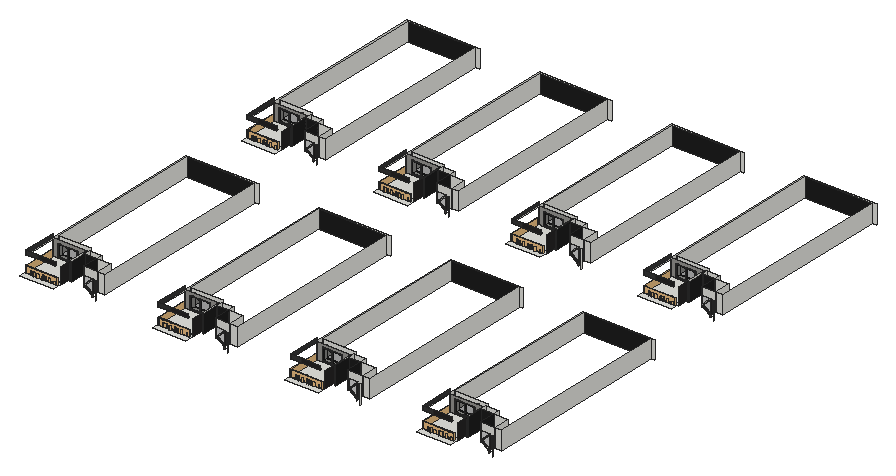
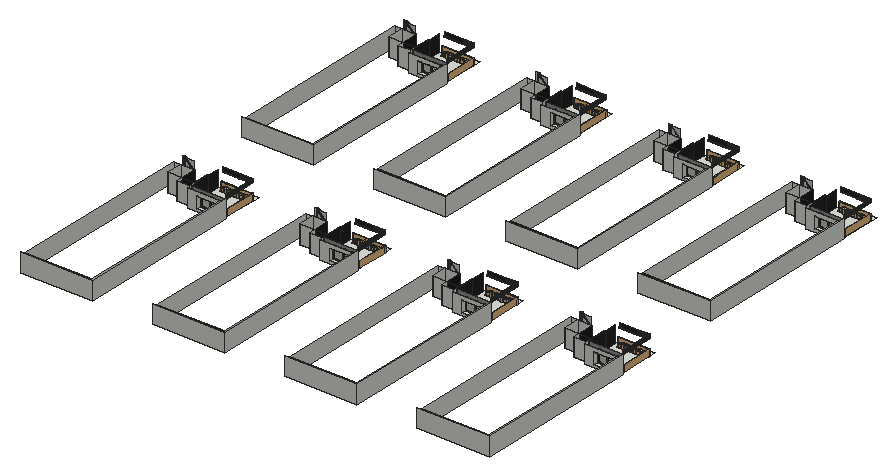
# SketchUp Ruby script. Lengths in inches.
U = 1.inch
M = Sketchup.active_model
def pt(a) = Geom::Point3d.new(a.map { |v| v * U })
def face(e, loops, mat)
  f = e.add_face(loops[0].map { |a| pt(a) })
  loops[1..].each { |l| e.add_face(l.map { |a| pt(a) }).erase! }
  f.material = f.back_material = mat if mat
  f
end
# faces: each face lists its corners as indices into pts; further lists are holes
def faces(e, pts, list, mat = nil) = list.each { |f| face(e, (f[0].is_a?(Array) ? f : [f]).map { |l| l.map { |i| pts[i] } }, mat) }
# xy, xz, yz: faces in a plane at the given z, y or x. An outline is a flat list of corners, or four numbers for a rectangle; further outlines are holes
def ring(l) = l.size == 4 ? [[l[0], l[1]], [l[2], l[1]], [l[2], l[3]], [l[0], l[3]]] : l.each_slice(2).to_a
def flat(e, list, mat, &to3) = list.each { |f| face(e, (f[0].is_a?(Array) ? f : [f]).map { |l| ring(l).map { |u, v| to3.(u, v) } }, mat) }
def xy(e, z, list, mat = nil) = flat(e, list, mat) { |x, y| [x, y, z] }
def xz(e, y, list, mat = nil) = flat(e, list, mat) { |x, z| [x, y, z] }
def yz(e, x, list, mat = nil) = flat(e, list, mat) { |y, z| [x, y, z] }
def lines(e, pts, list) = list.each { |a, b| e.add_line(pt(pts[a]), pt(pts[b])) }
# prism: a flat outline (further loops are holes) pulled along v
def prism(e, loops, v, mat = nil)
  f = face(e, loops, mat); d = Geom::Vector3d.new(v.map { |x| x * U })
  f.pushpull(f.normal.samedirection?(d) ? d.length : -d.length)
end
def box(e, o, s, mat = nil) = prism(e, [[o, [o[0] + s[0], o[1], o[2]], [o[0] + s[0], o[1] + s[1], o[2]], [o[0], o[1] + s[1], o[2]]]], [0, 0, s[2]], mat)
def at(x, y, z, deg = 0) = Geom::Transformation.translation(pt([x, y, z])) * Geom::Transformation.rotation(ORIGIN, Z_AXIS, deg.degrees)
def axes(o, x, y, z) = Geom::Transformation.new([*x, 0, *y, 0, *z, 0, *pt(o).to_a, 1])
def part(name) = M.definitions.add(name)
# library, detail: a bought-in or finely detailed component or shape, given as its bounding box
def library(name, o, s) = part(name).tap { |d| box(d.entities, o, s) }
def detail(e, o, s) = box(e.add_group.entities, o, s)
def put(e, d, t, mat = nil) = e.add_instance(d, t).tap { |i| i.material = mat if mat }
def group(e, t, mat = nil) = e.add_group.tap { |g| g.transformation = t; g.material = mat if mat }.entities
root = M.entities
M.materials.add("Glass_Tinted_Gray").color = [0, 0, 0]
M.materials["Glass_Tinted_Gray"].alpha = 0.125
M.materials.add("Material__1").color = [95, 70, 46]
M.materials.add("[0135_DarkGray]").color = [81, 81, 81]
M.materials.add("[Carrera Marble]").color = [207, 207, 207]
M.materials.add("[Color M06]").color = [86, 86, 86]
M.materials.add("[Color M08]").color = [30, 30, 30]
M.materials.add("[Field Square Tile]").color = [211, 167, 108]
M.materials.add("[Granite Dark Gray]").color = [38, 37, 37]
M.materials.add("[Granite Light Gray]").color = [149, 148, 144]
M.materials.add("[Granite Tile]1").color = [68, 65, 63]
M.materials.add("[Mirror 02]").color = [229, 229, 229]
M.materials.add("[Slate Light Tile]").color = [54, 54, 54]
M.materials.add("[Terrazzo Light Blue]").color = [196, 214, 227]
c1 = library("Areca palm plant",[0,0,0],[49.1,36.6,54.46])
c2 = library("Group\#74",[-84.69,-90.07,-0.36],[176.51,175.13,171.4])
c3 = library("Group38\#2",[14.01,28.44,-23.43],[18.58,18.32,38.89])
c4 = library("Group\#130",[-7.34,-1.2,0],[38.67,35.81,49.04])
c5 = library("Group20\#1",[-20.81,-17.08,3.79],[39.86,39.43,37.51])
c6 = part("Group\#3")
xy(c6.entities,0,[[0,0,6,234.8],[30,0,36,234.8]])
xy(c6.entities,3,[[6,0,30,234.8]])
xy(c6.entities,7,[[6,5,30,229.8]],"Material__1")
xy(c6.entities,15,[[[0,0,36,234.8],[6,5,30,229.8]]])
xz(c6.entities,0,[[0,0,6,0,6,3,30,3,30,0,36,0,36,15,0,15]])
xz(c6.entities,5,[[6,7,30,15]])
xz(c6.entities,229.8,[[6,7,30,15]])
xz(c6.entities,234.8,[[0,0,0,15,36,15,36,0,30,0,30,3,6,3,6,0]])
yz(c6.entities,0,[[0,0,234.8,15]])
yz(c6.entities,6,[[0,0,234.8,3],[5,7,229.8,15]])
yz(c6.entities,30,[[0,0,234.8,3],[5,7,229.8,15]])
yz(c6.entities,36,[[0,0,234.8,15]])
c7 = part("Group\#5")
put(c7.entities,c1,axes([-6.2,158.41,6.08],[0.45017,-0.56191,0],[0.66137,0.52986,0],[0,0,0.72]))
put(c7.entities,c1,axes([-6.2,56.6,6.08],[0.45017,-0.56191,0],[0.66137,0.52986,0],[0,0,0.72]))
put(c7.entities,c2,axes([17.19,15.79,6.07],[-0.08133,-0.14087,0],[0.14087,-0.08133,0],[0,0,0.1725]))
put(c7.entities,c2,axes([14.93,173.12,6.05],[-0.04961,-0.08593,0],[0.08593,-0.04961,0],[0,0,0.10522]))
put(c7.entities,c2,axes([17.19,223.04,6.07],[-0.08133,-0.14087,0],[0.14087,-0.08133,0],[0,0,0.1725]))
put(c7.entities,c3,axes([-4.1,-1.15,28.17],[0.8848,0,0],[0,0.94674,0],[0,0,0.85826]))
put(c7.entities,c2,axes([14.93,193.18,6.05],[-0.04961,-0.08593,0],[0.08593,-0.04961,0],[0,0,0.10522]))
put(c7.entities,c2,axes([14.93,91.37,6.05],[-0.04961,-0.08593,0],[0.08593,-0.04961,0],[0,0,0.10522]))
put(c7.entities,c4,axes([24.9375,191.72,8],[0,0.79,0],[-0.79,0,0],[0,0,0.79]))
put(c7.entities,c5,axes([18.97,181.79,4.77],[0,0.85,0],[-0.85,0,0],[0,0,0.85]))
put(c7.entities,c2,axes([14.93,145.87,6.05],[-0.04961,-0.08593,0],[0.08593,-0.04961,0],[0,0,0.10522]))
put(c7.entities,c5,axes([18.97,79.98,4.77],[0,0.85,0],[-0.85,0,0],[0,0,0.85]))
put(c7.entities,c2,axes([14.93,71.3,6.05],[-0.04961,-0.08593,0],[0.08593,-0.04961,0],[0,0,0.10522]))
put(c7.entities,c4,axes([24.9375,89.91,8],[0,0.79,0],[-0.79,0,0],[0,0,0.79]))
put(c7.entities,c2,axes([14.93,44.05,6.05],[-0.04961,-0.08593,0],[0.08593,-0.04961,0],[0,0,0.10522]))
put(c7.entities,c2,axes([17.19,121.23,6.07],[-0.08133,-0.14087,0],[0.14087,-0.08133,0],[0,0,0.1725]))
put(c7.entities,c6,at(0,0,0))
put(c7.entities,c3,axes([-4.1,100.66,28.17],[0.8848,0,0],[0,0.94674,0],[0,0,0.85826]))
c8 = library("Glass Railing",[0,0,0],[139.5,4.76,42])
c9 = part("PENTEK_RP Fineline 50S_Sliding_DoorCase_E1")
box(c9.entities,[0,0,0],[1.51,3.66,99.27],"[0135_DarkGray]")
c10 = part("PENTEK_RP Fineline 50S_SlidingDooe_Case_E2")
box(c10.entities,[0,0,0],[96.25,3.66,1.51],"[0135_DarkGray]")
c11 = part("pentek_RP Fineline 50S_SlidingDoor_Case")
put(c11.entities,c9,at(97.76,0,0))
put(c11.entities,c10,at(1.51,0,0))
put(c11.entities,c9,at(0,0,0))
put(c11.entities,c10,at(1.51,0,97.76))
c12 = part("PENTEK_RP Fineline 50S_SlidingDoor_GlazingBead_2")
box(c12.entities,[0,0,0],[0.56,0.59,94.39],"[0135_DarkGray]")
c13 = part("PENTEK_RP Fineline 50S_SlidingDoor_Glass")
box(c13.entities,[0,0,0],[46.58,0.16,94.39],"Glass_Tinted_Gray")
c14 = part("PENTEK_RP Fineline 50S_SlidingDoor_GlazingBead")
box(c14.entities,[0,0,0],[45.47,0.59,0.56],"[0135_DarkGray]")
c15 = part("PENTEK_RP Fineline 50S_SlidingDoor_Leaf_E1")
xy(c15.entities,0,[[0,0,0.93,1.97],[0.93,1.57,1.49,1.97]],"[0135_DarkGray]")
xy(c15.entities,96.25,[[0,0,0.93,0,0.93,1.57,1.49,1.57,1.49,1.97,0,1.97]],"[0135_DarkGray]")
xz(c15.entities,0,[[0,0,0.93,96.25]],"[0135_DarkGray]")
xz(c15.entities,1.57,[[0.93,0,1.49,95.32],[0.93,95.32,1.49,96.25]],"[0135_DarkGray]")
xz(c15.entities,1.97,[[0,0,1.49,96.25]],"[0135_DarkGray]")
yz(c15.entities,0,[[0,0,1.97,96.25]],"[0135_DarkGray]")
yz(c15.entities,0.93,[[0,0,1.57,0.93],[0,0.93,1.57,95.32],[0,95.32,1.57,96.25]],"[0135_DarkGray]")
yz(c15.entities,1.49,[[1.57,0,1.97,95.32],[1.57,95.32,1.97,96.25]],"[0135_DarkGray]")
c16 = part("PENTEK_RP Fineline 50S_SlidingDoor_Leaf_E2")
xy(c16.entities,0,[[0,0,0,1.57,0.56,1.57,0.56,1.97,46.02,1.97,46.02,1.57,46.58,1.57,46.58,0]],"[0135_DarkGray]")
xy(c16.entities,0.93,[[0,0,46.58,1.57]],"[0135_DarkGray]")
xy(c16.entities,1.49,[[0.56,1.57,46.02,1.97]],"[0135_DarkGray]")
xz(c16.entities,0,[[0,0,46.58,0.93]],"[0135_DarkGray]")
xz(c16.entities,1.57,[[0,0,0.56,0.93],[46.02,0,46.58,0.93],[0.56,0.93,46.02,1.49]],"[0135_DarkGray]")
xz(c16.entities,1.97,[[0.56,0,46.02,1.49]],"[0135_DarkGray]")
yz(c16.entities,0,[[0,0,1.57,0.93]],"[0135_DarkGray]")
yz(c16.entities,0.56,[[1.57,0,1.97,0.93],[1.57,0.93,1.97,1.49]],"[0135_DarkGray]")
yz(c16.entities,46.02,[[1.57,0,1.97,0.93],[1.57,0.93,1.97,1.49]],"[0135_DarkGray]")
yz(c16.entities,46.58,[[0,0,1.57,0.93]],"[0135_DarkGray]")
c17 = part("PENTEK_RP Fineline S_SlidingDoor_Leaf1")
put(c17.entities,c12,at(0.93,0,0.93))
put(c17.entities,c12,at(46.96,0,0.93))
put(c17.entities,c13,at(1.49,1.42,0.93))
put(c17.entities,c14,at(1.49,0,0.93))
put(c17.entities,c13,at(1.49,0.59,0.93),"[Terrazzo Light Blue]")
put(c17.entities,c15,at(0,0,0))
put(c17.entities,c15,axes([48.44,0,0],[-1,0,0],[0,1,0],[0,0,1]))
put(c17.entities,c16,axes([0.93,0,96.25],[1,0,0],[0,1,0],[0,0,-1]))
put(c17.entities,c16,at(0.93,0,0))
put(c17.entities,c14,at(1.49,0,94.77))
c18 = part("PENTEK_RP Fineline 50S_SlidingDoor_Leaf2")
put(c18.entities,c13,at(1.49,1.42,0.93))
put(c18.entities,c14,at(1.49,0,94.77))
put(c18.entities,c12,at(46.96,0,0.93))
put(c18.entities,c13,at(1.49,0.59,0.93),"[Mirror 02]")
put(c18.entities,c12,at(0.93,0,0.93))
put(c18.entities,c15,at(0,0,0))
put(c18.entities,c15,axes([48.44,0,0],[-1,0,0],[0,1,0],[0,0,1]))
put(c18.entities,c14,at(1.49,0,0.93))
put(c18.entities,c16,axes([0.93,0,96.25],[1,0,0],[0,1,0],[0,0,-1]))
put(c18.entities,c16,at(0.93,0,0))
c19 = part("PENTEK - Slimmest Steel Sliding Door / Window\#1")
put(c19.entities,c11,at(0,-1.88,-0.09))
put(c19.entities,c17,at(1.51,-2.27,1.42))
put(c19.entities,c18,at(49.32,-0.3,1.42))
xy(root,260.5,[[445.08,589.83,453.7,697.21],[534.46,589.83,629.77,697.21],[1323.83,589.83,1332.45,697.21],[1413.21,589.83,1508.52,697.21],[2202.58,589.83,2211.2,697.21],
  [2291.96,589.83,2387.27,697.21],[3081.33,589.83,3089.95,697.21],[3170.71,589.83,3266.02,697.21],[445.08,2425.46,453.7,2532.83],[534.46,2425.46,629.77,2532.83],
  [1323.83,2425.46,1332.45,2532.83],[1413.21,2425.46,1508.52,2532.83],[2202.58,2425.46,2211.2,2532.83],[2291.96,2425.46,2387.27,2532.83],[3081.33,2425.46,3089.95,2532.83],
  [3170.71,2425.46,3266.02,2532.83]])
xy(root,260.5,[[453.7,697.21,534.46,738.02],[1332.45,697.21,1413.21,738.02],[2211.2,697.21,2291.96,738.02],[3089.95,697.21,3170.71,738.02],[453.7,2532.83,534.46,2573.65],
  [1332.45,2532.83,1413.21,2573.65],[2211.2,2532.83,2291.96,2573.65],[3089.95,2532.83,3170.71,2573.65]],"[Color M08]")
xy(root,270.8125,[[218.97,458.5,442.35,458.5,442.35,511.08,444.78,511.08,444.78,727.2,218.97,727.2],[1097.72,458.5,1321.1,458.5,1321.1,511.08,1323.53,511.08,1323.53,727.2,1097.72,727.2],[1976.47,458.5,2199.85,458.5,2199.85,511.08,2202.28,511.08,2202.28,727.2,1976.47,727.2],[2855.22,458.5,3078.6,458.5,3078.6,511.08,3081.03,511.08,3081.03,727.2,2855.22,727.2],[218.97,2294.125,442.35,2294.125,442.35,2346.71,444.78,2346.71,444.78,2562.82,218.97,2562.82],
  [1097.72,2294.125,1321.1,2294.125,1321.1,2346.71,1323.53,2346.71,1323.53,2562.82,1097.72,2562.82],[1976.47,2294.125,2199.85,2294.125,2199.85,2346.71,2202.28,2346.71,2202.28,2562.82,1976.47,2562.82],[2855.22,2294.125,3078.6,2294.125,3078.6,2346.71,3081.03,2346.71,3081.03,2562.82,2855.22,2562.82]])
xy(root,276.7,[[254.08,727.2,382.72,762.17],[1132.83,727.2,1261.47,762.17],[2011.58,727.2,2140.22,762.17],[2890.33,727.2,3018.97,762.17],[254.08,2562.82,382.72,2597.8],
  [1132.83,2562.82,1261.47,2597.8],[2011.58,2562.82,2140.22,2597.8],[2890.33,2562.82,3018.97,2597.8]])
xy(root,282.18,[[659.68,501.4,665.11,508.33],[1538.43,501.4,1543.86,508.33],[2417.18,501.4,2422.61,508.33],[3295.93,501.4,3301.36,508.33],[659.68,2337.02,665.11,2343.96],
  [1538.43,2337.02,1543.86,2343.96],[2417.18,2337.02,2422.61,2343.96],[3295.93,2337.02,3301.36,2343.96]],"[Granite Dark Gray]")
xy(root,296.03,[[659.68,501.4,665.11,508.33],[1538.43,501.4,1543.86,508.33],[2417.18,501.4,2422.61,508.33],[3295.93,501.4,3301.36,508.33],[659.68,2337.02,665.11,2343.96],
  [1538.43,2337.02,1543.86,2343.96],[2417.18,2337.02,2422.61,2343.96],[3295.93,2337.02,3301.36,2343.96]],"[Granite Dark Gray]")
xy(root,356.2,[[254.08,727.2,382.72,762.17],[1132.83,727.2,1261.47,762.17],[2011.58,727.2,2140.22,762.17],[2890.33,727.2,3018.97,762.17],[254.08,2562.82,382.72,2597.8],
  [1132.83,2562.82,1261.47,2597.8],[2011.58,2562.82,2140.22,2597.8],[2890.33,2562.82,3018.97,2597.8]])
xy(root,376.5,[[218.97,504.52,218.97,727.2,223.8,727.2,223.8,512.27,295.73,512.27,295.73,504.52],[1097.72,504.52,1097.72,727.2,1102.55,727.2,1102.55,512.27,1174.48,512.27,1174.48,504.52],[1976.47,504.52,1976.47,727.2,1981.3,727.2,1981.3,512.27,2053.23,512.27,2053.23,504.52],[2855.22,504.52,2855.22,727.2,2860.05,727.2,2860.05,512.27,2931.98,512.27,2931.98,504.52],[218.97,2340.15,218.97,2562.82,223.8,2562.82,223.8,2347.9,295.73,2347.9,295.73,2340.15],
  [1097.72,2340.15,1097.72,2562.82,1102.55,2562.82,1102.55,2347.9,1174.48,2347.9,1174.48,2340.15],[1976.47,2340.15,1976.47,2562.82,1981.3,2562.82,1981.3,2347.9,2053.23,2347.9,2053.23,2340.15],[2855.22,2340.15,2855.22,2562.82,2860.05,2562.82,2860.05,2347.9,2931.98,2347.9,2931.98,2340.15]],"[Color M06]")
xy(root,376.5,[[295.73,504.52,414.98,512.27],[1174.48,504.52,1293.73,512.27],[2053.23,504.52,2172.48,512.27],[2931.98,504.52,3051.23,512.27],[295.73,2340.15,414.98,2347.9],
  [1174.48,2340.15,1293.73,2347.9],[2053.23,2340.15,2172.48,2347.9],[2931.98,2340.15,3051.23,2347.9]],"[Granite Dark Gray]")
xz(root,501.4,[[659.68,282.18,665.11,296.03],[1538.43,282.18,1543.86,296.03],[2417.18,282.18,2422.61,296.03],[3295.93,282.18,3301.36,296.03]],"[Granite Tile]1")
xz(root,504.52,[[295.73,376.5,414.98,403.8125],[1174.48,376.5,1293.73,403.8125],[2053.23,376.5,2172.48,403.8125],[2931.98,376.5,3051.23,403.8125]],"[Granite Dark Gray]")
xz(root,504.52,[[218.97,376.5,295.73,403.8125],[1097.72,376.5,1174.48,403.8125],[1976.47,376.5,2053.23,403.8125],[2855.22,376.5,2931.98,403.8125]],"[Slate Light Tile]")
xz(root,508.33,[[659.68,296.03,665.11,380.5],[1538.43,296.03,1543.86,380.5],[2417.18,296.03,2422.61,380.5],[3295.93,296.03,3301.36,380.5]],"[Granite Dark Gray]")
xz(root,511.08,[[676.54,260.5,677.98,380.5],[1555.29,260.5,1556.73,380.5],[2434.04,260.5,2435.48,380.5],[3312.79,260.5,3314.23,380.5]])
xz(root,512.27,[[223.8,376.5,295.73,380.5],[295.73,376.5,414.98,380.5],[1102.55,376.5,1174.48,380.5],[1174.48,376.5,1293.73,380.5],[1981.3,376.5,2053.23,380.5],
  [2053.23,376.5,2172.48,380.5],[2860.05,376.5,2931.98,380.5],[2931.98,376.5,3051.23,380.5]])
xz(root,513.52,[[653.06,284.38,653.06,290.71,605.1875,327.66,653.06,374,653.06,380.5,599.51,327.51],[1531.81,284.38,1531.81,290.71,1483.9375,327.66,1531.81,374,1531.81,380.5,1478.26,327.51],[2410.56,284.38,2410.56,290.71,2362.6875,327.66,2410.56,374,2410.56,380.5,2357.01,327.51],[3289.31,284.38,3289.31,290.71,3241.4375,327.66,3289.31,374,3289.31,380.5,3235.76,327.51]],"[Field Square Tile]")
xz(root,518.65,[[653.06,290.71,653.06,374,605.1875,327.66],[1531.81,290.71,1531.81,374,1483.9375,327.66],[2410.56,290.71,2410.56,374,2362.6875,327.66],[3289.31,290.71,3289.31,374,3241.4375,327.66],[599.51,327.51,653.06,380.5,599.51,380.5],
  [1478.26,327.51,1531.81,380.5,1478.26,380.5],[2357.01,327.51,2410.56,380.5,2357.01,380.5],[3235.76,327.51,3289.31,380.5,3235.76,380.5]],"[Carrera Marble]")
xz(root,589.83,[[444.78,260.5,445.08,380.5],[445.08,260.5,453.7,380.5],[534.46,260.5,629.77,380.5],[629.77,260.5,676.54,380.5],[1323.53,260.5,1323.83,380.5],
  [1323.83,260.5,1332.45,380.5],[1413.21,260.5,1508.52,380.5],[1508.52,260.5,1555.29,380.5],[2202.28,260.5,2202.58,380.5],[2202.58,260.5,2211.2,380.5],
  [2291.96,260.5,2387.27,380.5],[2387.27,260.5,2434.04,380.5],[3081.03,260.5,3081.33,380.5],[3081.33,260.5,3089.95,380.5],[3170.71,260.5,3266.02,380.5],
  [3266.02,260.5,3312.79,380.5]])
xz(root,697.21,[[445.08,260.5,453.7,380.5],[534.46,260.5,629.77,380.5],[1323.83,260.5,1332.45,380.5],[1413.21,260.5,1508.52,380.5],[2202.58,260.5,2211.2,380.5],
  [2291.96,260.5,2387.27,380.5],[3081.33,260.5,3089.95,380.5],[3170.71,260.5,3266.02,380.5]])
xz(root,697.21,[[453.7,260.5,534.46,380.5],[1332.45,260.5,1413.21,380.5],[2211.2,260.5,2291.96,380.5],[3089.95,260.5,3170.71,380.5]],"[Color M08]")
xz(root,727.2,[[218.97,376.5,223.8,380.5],[1097.72,376.5,1102.55,380.5],[1976.47,376.5,1981.3,380.5],[2855.22,376.5,2860.05,380.5]])
xz(root,727.2,[[218.97,270.8125,254.08,270.8125,254.08,356.2,382.72,356.2,382.72,276.7,254.08,276.7,254.08,270.8125,444.78,270.8125,444.78,380.5,223.8,380.5,223.8,376.5,218.97,376.5],[1097.72,270.8125,1132.83,270.8125,1132.83,356.2,1261.47,356.2,1261.47,276.7,1132.83,276.7,1132.83,270.8125,1323.53,270.8125,1323.53,380.5,1102.55,380.5,1102.55,376.5,1097.72,376.5],[1976.47,270.8125,2011.58,270.8125,2011.58,356.2,2140.22,356.2,2140.22,276.7,2011.58,276.7,2011.58,270.8125,2202.28,270.8125,2202.28,380.5,1981.3,380.5,1981.3,376.5,1976.47,376.5],[2855.22,270.8125,2890.33,270.8125,2890.33,356.2,3018.97,356.2,3018.97,276.7,2890.33,276.7,2890.33,270.8125,3081.03,270.8125,3081.03,380.5,2860.05,380.5,2860.05,376.5,2855.22,376.5]],"[Granite Light Gray]")
xz(root,738.02,[[453.7,260.5,534.46,380.5],[1332.45,260.5,1413.21,380.5],[2211.2,260.5,2291.96,380.5],[3089.95,260.5,3170.71,380.5]])
xz(root,762.17,[[[228.78,260.5,444.78,380.5],[254.08,276.7,382.72,356.2]],[[1107.53,260.5,1323.53,380.5],[1132.83,276.7,1261.47,356.2]],[[1986.28,260.5,2202.28,380.5],[2011.58,276.7,2140.22,356.2]],[[2865.03,260.5,3081.03,380.5],[2890.33,276.7,3018.97,356.2]]])
xz(root,1825.82,[[228.78,260.5,676.54,380.5],[1107.53,260.5,1555.29,380.5],[1986.28,260.5,2434.04,380.5],[2865.03,260.5,3312.79,380.5]],"[Color M08]")
xz(root,1835.625,[[218.97,260.5,698.16,380.5],[1097.72,260.5,1576.91,380.5],[1976.47,260.5,2455.66,380.5],[2855.22,260.5,3334.41,380.5]])
xz(root,2337.02,[[659.68,282.18,665.11,296.03],[1538.43,282.18,1543.86,296.03],[2417.18,282.18,2422.61,296.03],[3295.93,282.18,3301.36,296.03]],"[Granite Tile]1")
xz(root,2340.15,[[295.73,376.5,414.98,403.8125],[1174.48,376.5,1293.73,403.8125],[2053.23,376.5,2172.48,403.8125],[2931.98,376.5,3051.23,403.8125]],"[Granite Dark Gray]")
xz(root,2340.15,[[218.97,376.5,295.73,403.8125],[1097.72,376.5,1174.48,403.8125],[1976.47,376.5,2053.23,403.8125],[2855.22,376.5,2931.98,403.8125]],"[Slate Light Tile]")
xz(root,2343.96,[[659.68,296.03,665.11,380.5],[1538.43,296.03,1543.86,380.5],[2417.18,296.03,2422.61,380.5],[3295.93,296.03,3301.36,380.5]],"[Granite Dark Gray]")
xz(root,2346.71,[[676.54,260.5,677.98,380.5],[1555.29,260.5,1556.73,380.5],[2434.04,260.5,2435.48,380.5],[3312.79,260.5,3314.23,380.5]])
xz(root,2347.9,[[223.8,376.5,295.73,380.5],[295.73,376.5,414.98,380.5],[1102.55,376.5,1174.48,380.5],[1174.48,376.5,1293.73,380.5],[1981.3,376.5,2053.23,380.5],
  [2053.23,376.5,2172.48,380.5],[2860.05,376.5,2931.98,380.5],[2931.98,376.5,3051.23,380.5]])
xz(root,2349.15,[[653.06,284.38,653.06,290.71,605.1875,327.66,653.06,374,653.06,380.5,599.51,327.51],[1531.81,284.38,1531.81,290.71,1483.9375,327.66,1531.81,374,1531.81,380.5,1478.26,327.51],[2410.56,284.38,2410.56,290.71,2362.6875,327.66,2410.56,374,2410.56,380.5,2357.01,327.51],[3289.31,284.38,3289.31,290.71,3241.4375,327.66,3289.31,374,3289.31,380.5,3235.76,327.51]],"[Field Square Tile]")
xz(root,2354.27,[[653.06,290.71,653.06,374,605.1875,327.66],[1531.81,290.71,1531.81,374,1483.9375,327.66],[2410.56,290.71,2410.56,374,2362.6875,327.66],[3289.31,290.71,3289.31,374,3241.4375,327.66],[599.51,327.51,653.06,380.5,599.51,380.5],
  [1478.26,327.51,1531.81,380.5,1478.26,380.5],[2357.01,327.51,2410.56,380.5,2357.01,380.5],[3235.76,327.51,3289.31,380.5,3235.76,380.5]],"[Carrera Marble]")
xz(root,2425.46,[[444.78,260.5,445.08,380.5],[445.08,260.5,453.7,380.5],[534.46,260.5,629.77,380.5],[629.77,260.5,676.54,380.5],[1323.53,260.5,1323.83,380.5],
  [1323.83,260.5,1332.45,380.5],[1413.21,260.5,1508.52,380.5],[1508.52,260.5,1555.29,380.5],[2202.28,260.5,2202.58,380.5],[2202.58,260.5,2211.2,380.5],
  [2291.96,260.5,2387.27,380.5],[2387.27,260.5,2434.04,380.5],[3081.03,260.5,3081.33,380.5],[3081.33,260.5,3089.95,380.5],[3170.71,260.5,3266.02,380.5],
  [3266.02,260.5,3312.79,380.5]])
xz(root,2532.83,[[445.08,260.5,453.7,380.5],[534.46,260.5,629.77,380.5],[1323.83,260.5,1332.45,380.5],[1413.21,260.5,1508.52,380.5],[2202.58,260.5,2211.2,380.5],
  [2291.96,260.5,2387.27,380.5],[3081.33,260.5,3089.95,380.5],[3170.71,260.5,3266.02,380.5]])
xz(root,2532.83,[[453.7,260.5,534.46,380.5],[1332.45,260.5,1413.21,380.5],[2211.2,260.5,2291.96,380.5],[3089.95,260.5,3170.71,380.5]],"[Color M08]")
xz(root,2562.82,[[218.97,376.5,223.8,380.5],[1097.72,376.5,1102.55,380.5],[1976.47,376.5,1981.3,380.5],[2855.22,376.5,2860.05,380.5]])
xz(root,2562.82,[[218.97,270.8125,254.08,270.8125,254.08,356.2,382.72,356.2,382.72,276.7,254.08,276.7,254.08,270.8125,444.78,270.8125,444.78,380.5,223.8,380.5,223.8,376.5,218.97,376.5],[1097.72,270.8125,1132.83,270.8125,1132.83,356.2,1261.47,356.2,1261.47,276.7,1132.83,276.7,1132.83,270.8125,1323.53,270.8125,1323.53,380.5,1102.55,380.5,1102.55,376.5,1097.72,376.5],[1976.47,270.8125,2011.58,270.8125,2011.58,356.2,2140.22,356.2,2140.22,276.7,2011.58,276.7,2011.58,270.8125,2202.28,270.8125,2202.28,380.5,1981.3,380.5,1981.3,376.5,1976.47,376.5],[2855.22,270.8125,2890.33,270.8125,2890.33,356.2,3018.97,356.2,3018.97,276.7,2890.33,276.7,2890.33,270.8125,3081.03,270.8125,3081.03,380.5,2860.05,380.5,2860.05,376.5,2855.22,376.5]],"[Granite Light Gray]")
xz(root,2573.65,[[453.7,260.5,534.46,380.5],[1332.45,260.5,1413.21,380.5],[2211.2,260.5,2291.96,380.5],[3089.95,260.5,3170.71,380.5]])
xz(root,2597.8,[[[228.78,260.5,444.78,380.5],[254.08,276.7,382.72,356.2]],[[1107.53,260.5,1323.53,380.5],[1132.83,276.7,1261.47,356.2]],[[1986.28,260.5,2202.28,380.5],[2011.58,276.7,2140.22,356.2]],[[2865.03,260.5,3081.03,380.5],[2890.33,276.7,3018.97,356.2]]])
xz(root,3661.44,[[228.78,260.5,676.54,380.5],[1107.53,260.5,1555.29,380.5],[1986.28,260.5,2434.04,380.5],[2865.03,260.5,3312.79,380.5]],"[Color M08]")
xz(root,3671.25,[[218.97,260.5,698.16,380.5],[1097.72,260.5,1576.91,380.5],[1976.47,260.5,2455.66,380.5],[2855.22,260.5,3334.41,380.5]])
yz(root,218.97,[[727.2,260.5,1835.625,380.5],[2562.82,260.5,3671.25,380.5]])
yz(root,218.97,[[504.52,376.5,727.2,403.8125],[2340.15,376.5,2562.82,403.8125]],"[Slate Light Tile]")
yz(root,223.8,[[512.27,376.5,727.2,380.5],[2347.9,376.5,2562.82,380.5]])
yz(root,228.78,[[762.17,260.5,1825.82,380.5],[2597.8,260.5,3661.44,380.5]])
yz(root,254.08,[[727.2,276.7,762.17,356.2],[2562.82,276.7,2597.8,356.2]])
yz(root,382.72,[[727.2,276.7,762.17,356.2],[2562.82,276.7,2597.8,356.2]])
yz(root,414.98,[[504.52,376.5,512.27,380.5],[2340.15,376.5,2347.9,380.5]],"[Granite Dark Gray]")
yz(root,444.78,[[511.08,270.8125,589.83,380.5],[589.83,270.8125,727.2,380.5],[2346.71,270.8125,2425.46,380.5],[2425.46,270.8125,2562.82,380.5]],"[Granite Dark Gray]")
yz(root,445.08,[[589.83,260.5,697.21,380.5],[2425.46,260.5,2532.83,380.5]])
yz(root,453.7,[[697.21,260.5,738.02,380.5],[2532.83,260.5,2573.65,380.5]])
yz(root,453.7,[[589.83,260.5,697.21,380.5],[2425.46,260.5,2532.83,380.5]],"[Color M08]")
yz(root,534.46,[[697.21,260.5,738.02,380.5],[2532.83,260.5,2573.65,380.5]])
yz(root,534.46,[[589.83,260.5,697.21,380.5],[2425.46,260.5,2532.83,380.5]],"[Color M08]")
yz(root,629.77,[[589.83,260.5,697.21,380.5],[2425.46,260.5,2532.83,380.5]])
yz(root,676.54,[[589.83,260.5,1825.82,380.5],[2425.46,260.5,3661.44,380.5]])
yz(root,1097.72,[[727.2,260.5,1835.625,380.5],[2562.82,260.5,3671.25,380.5]])
yz(root,1097.72,[[504.52,376.5,727.2,403.8125],[2340.15,376.5,2562.82,403.8125]],"[Slate Light Tile]")
yz(root,1102.55,[[512.27,376.5,727.2,380.5],[2347.9,376.5,2562.82,380.5]])
yz(root,1107.53,[[762.17,260.5,1825.82,380.5],[2597.8,260.5,3661.44,380.5]])
yz(root,1132.83,[[727.2,276.7,762.17,356.2],[2562.82,276.7,2597.8,356.2]])
yz(root,1261.47,[[727.2,276.7,762.17,356.2],[2562.82,276.7,2597.8,356.2]])
yz(root,1293.73,[[504.52,376.5,512.27,380.5],[2340.15,376.5,2347.9,380.5]],"[Granite Dark Gray]")
yz(root,1323.53,[[511.08,270.8125,589.83,380.5],[589.83,270.8125,727.2,380.5],[2346.71,270.8125,2425.46,380.5],[2425.46,270.8125,2562.82,380.5]],"[Granite Dark Gray]")
yz(root,1323.83,[[589.83,260.5,697.21,380.5],[2425.46,260.5,2532.83,380.5]])
yz(root,1332.45,[[697.21,260.5,738.02,380.5],[2532.83,260.5,2573.65,380.5]])
yz(root,1332.45,[[589.83,260.5,697.21,380.5],[2425.46,260.5,2532.83,380.5]],"[Color M08]")
yz(root,1413.21,[[697.21,260.5,738.02,380.5],[2532.83,260.5,2573.65,380.5]])
yz(root,1413.21,[[589.83,260.5,697.21,380.5],[2425.46,260.5,2532.83,380.5]],"[Color M08]")
yz(root,1508.52,[[589.83,260.5,697.21,380.5],[2425.46,260.5,2532.83,380.5]])
yz(root,1555.29,[[589.83,260.5,1825.82,380.5],[2425.46,260.5,3661.44,380.5]])
yz(root,1976.47,[[727.2,260.5,1835.625,380.5],[2562.82,260.5,3671.25,380.5]])
yz(root,1976.47,[[504.52,376.5,727.2,403.8125],[2340.15,376.5,2562.82,403.8125]],"[Slate Light Tile]")
yz(root,1981.3,[[512.27,376.5,727.2,380.5],[2347.9,376.5,2562.82,380.5]])
yz(root,1986.28,[[762.17,260.5,1825.82,380.5],[2597.8,260.5,3661.44,380.5]])
yz(root,2011.58,[[727.2,276.7,762.17,356.2],[2562.82,276.7,2597.8,356.2]])
yz(root,2140.22,[[727.2,276.7,762.17,356.2],[2562.82,276.7,2597.8,356.2]])
yz(root,2172.48,[[504.52,376.5,512.27,380.5],[2340.15,376.5,2347.9,380.5]],"[Granite Dark Gray]")
yz(root,2202.28,[[511.08,270.8125,589.83,380.5],[589.83,270.8125,727.2,380.5],[2346.71,270.8125,2425.46,380.5],[2425.46,270.8125,2562.82,380.5]],"[Granite Dark Gray]")
yz(root,2202.58,[[589.83,260.5,697.21,380.5],[2425.46,260.5,2532.83,380.5]])
yz(root,2211.2,[[697.21,260.5,738.02,380.5],[2532.83,260.5,2573.65,380.5]])
yz(root,2211.2,[[589.83,260.5,697.21,380.5],[2425.46,260.5,2532.83,380.5]],"[Color M08]")
yz(root,2291.96,[[697.21,260.5,738.02,380.5],[2532.83,260.5,2573.65,380.5]])
yz(root,2291.96,[[589.83,260.5,697.21,380.5],[2425.46,260.5,2532.83,380.5]],"[Color M08]")
yz(root,2387.27,[[589.83,260.5,697.21,380.5],[2425.46,260.5,2532.83,380.5]])
yz(root,2434.04,[[589.83,260.5,1825.82,380.5],[2425.46,260.5,3661.44,380.5]])
yz(root,2855.22,[[727.2,260.5,1835.625,380.5],[2562.82,260.5,3671.25,380.5]])
yz(root,2855.22,[[504.52,376.5,727.2,403.8125],[2340.15,376.5,2562.82,403.8125]],"[Slate Light Tile]")
yz(root,2860.05,[[512.27,376.5,727.2,380.5],[2347.9,376.5,2562.82,380.5]])
yz(root,2865.03,[[762.17,260.5,1825.82,380.5],[2597.8,260.5,3661.44,380.5]])
yz(root,2890.33,[[727.2,276.7,762.17,356.2],[2562.82,276.7,2597.8,356.2]])
yz(root,3018.97,[[727.2,276.7,762.17,356.2],[2562.82,276.7,2597.8,356.2]])
yz(root,3051.23,[[504.52,376.5,512.27,380.5],[2340.15,376.5,2347.9,380.5]],"[Granite Dark Gray]")
yz(root,3081.03,[[511.08,270.8125,589.83,380.5],[589.83,270.8125,727.2,380.5],[2346.71,270.8125,2425.46,380.5],[2425.46,270.8125,2562.82,380.5]],"[Granite Dark Gray]")
yz(root,3081.33,[[589.83,260.5,697.21,380.5],[2425.46,260.5,2532.83,380.5]])
yz(root,3089.95,[[697.21,260.5,738.02,380.5],[2532.83,260.5,2573.65,380.5]])
yz(root,3089.95,[[589.83,260.5,697.21,380.5],[2425.46,260.5,2532.83,380.5]],"[Color M08]")
yz(root,3170.71,[[697.21,260.5,738.02,380.5],[2532.83,260.5,2573.65,380.5]])
yz(root,3170.71,[[589.83,260.5,697.21,380.5],[2425.46,260.5,2532.83,380.5]],"[Color M08]")
yz(root,3266.02,[[589.83,260.5,697.21,380.5],[2425.46,260.5,2532.83,380.5]])
yz(root,3312.79,[[589.83,260.5,1825.82,380.5],[2425.46,260.5,3661.44,380.5]])
p = [[599.51,518.65,327.51],[653.06,518.65,284.38],[653.06,513.52,284.38],[599.51,513.52,327.51],[1478.26,518.65,327.51],[1531.81,518.65,284.38],
  [1531.81,513.52,284.38],[1478.26,513.52,327.51],[2357.01,518.65,327.51],[2410.56,518.65,284.38],[2410.56,513.52,284.38],[2357.01,513.52,327.51],
  [3235.76,518.65,327.51],[3289.31,518.65,284.38],[3289.31,513.52,284.38],[3235.76,513.52,327.51],[599.51,2354.27,327.51],[653.06,2354.27,284.38],
  [653.06,2349.15,284.38],[599.51,2349.15,327.51],[1478.26,2354.27,327.51],[1531.81,2354.27,284.38],[1531.81,2349.15,284.38],[1478.26,2349.15,327.51],
  [2357.01,2354.27,327.51],[2410.56,2354.27,284.38],[2410.56,2349.15,284.38],[2357.01,2349.15,327.51],[3235.76,2354.27,327.51],[3289.31,2354.27,284.38],
  [3289.31,2349.15,284.38],[3235.76,2349.15,327.51],[653.06,518.65,290.71],[605.1875,518.65,327.66],[605.1875,513.52,327.66],[653.06,513.52,290.71],
  [1531.81,518.65,290.71],[1483.9375,518.65,327.66],[1483.9375,513.52,327.66],[1531.81,513.52,290.71],[2410.56,518.65,290.71],[2362.6875,518.65,327.66],
  [2362.6875,513.52,327.66],[2410.56,513.52,290.71],[3289.31,518.65,290.71],[3241.4375,518.65,327.66],[3241.4375,513.52,327.66],[3289.31,513.52,290.71],
  [653.06,2354.27,290.71],[605.1875,2354.27,327.66],[605.1875,2349.15,327.66],[653.06,2349.15,290.71],[1531.81,2354.27,290.71],[1483.9375,2354.27,327.66],
  [1483.9375,2349.15,327.66],[1531.81,2349.15,290.71],[2410.56,2354.27,290.71],[2362.6875,2354.27,327.66],[2362.6875,2349.15,327.66],[2410.56,2349.15,290.71],
  [3289.31,2354.27,290.71],[3241.4375,2354.27,327.66],[3241.4375,2349.15,327.66],[3289.31,2349.15,290.71],[653.06,518.65,380.5],[653.06,513.52,380.5],
  [1531.81,518.65,380.5],[1531.81,513.52,380.5],[2410.56,518.65,380.5],[2410.56,513.52,380.5],[3289.31,518.65,380.5],[3289.31,513.52,380.5],
  [653.06,2354.27,380.5],[653.06,2349.15,380.5],[1531.81,2354.27,380.5],[1531.81,2349.15,380.5],[2410.56,2354.27,380.5],[2410.56,2349.15,380.5],
  [3289.31,2354.27,380.5],[3289.31,2349.15,380.5],[653.06,518.65,374],[653.06,513.52,374],[1531.81,518.65,374],[1531.81,513.52,374],
  [2410.56,518.65,374],[2410.56,513.52,374],[3289.31,518.65,374],[3289.31,513.52,374],[653.06,2354.27,374],[653.06,2349.15,374],
  [1531.81,2354.27,374],[1531.81,2349.15,374],[2410.56,2354.27,374],[2410.56,2349.15,374],[3289.31,2354.27,374],[3289.31,2349.15,374]]
faces(root,p,[[0,1,2,3],[4,5,6,7],[8,9,10,11],[12,13,14,15],[16,17,18,19],[20,21,22,23],[24,25,26,27],[28,29,30,31],
  [32,33,34,35],[36,37,38,39],[40,41,42,43],[44,45,46,47],[48,49,50,51],[52,53,54,55],[56,57,58,59],[60,61,62,63],
  [64,0,3,65],[66,4,7,67],[68,8,11,69],[70,12,15,71],[72,16,19,73],[74,20,23,75],[76,24,27,77],[78,28,31,79],
  [33,80,81,34],[37,82,83,38],[41,84,85,42],[45,86,87,46],[49,88,89,50],[53,90,91,54],[57,92,93,58],[61,94,95,62]])
put(root,c7,axes([2175.02,501.91,260.14],[0,0.7469,0],[-0.7469,0,0],[0,0,0.7469]))
put(root,c7,axes([3053.77,501.91,260.14],[0,0.7469,0],[-0.7469,0,0],[0,0,0.7469]))
put(root,c7,axes([1296.27,501.91,260.14],[0,0.7469,0],[-0.7469,0,0],[0,0,0.7469]))
put(root,c7,axes([417.52,501.91,260.14],[0,0.7469,0],[-0.7469,0,0],[0,0,0.7469]))
put(root,c7,axes([3053.77,2337.54,260.14],[0,0.7469,0],[-0.7469,0,0],[0,0,0.7469]))
put(root,c7,axes([2175.02,2337.54,260.14],[0,0.7469,0],[-0.7469,0,0],[0,0,0.7469]))
put(root,c7,axes([417.52,2337.54,260.14],[0,0.7469,0],[-0.7469,0,0],[0,0,0.7469]))
put(root,c7,axes([1296.27,2337.54,260.14],[0,0.7469,0],[-0.7469,0,0],[0,0,0.7469]))
put(root,c8,axes([1976.3,501.72,270.8125],[1.51,0,0],[0,1,0],[0,0,1]),"[Color M08]")
put(root,c8,axes([1976.47,712.37,270.8125],[0,-1.51,0],[1,0,0],[0,0,1]))
put(root,c8,axes([2855.22,712.37,270.8125],[0,-1.51,0],[1,0,0],[0,0,1]))
put(root,c8,axes([2855.05,501.72,270.8125],[1.51,0,0],[0,1,0],[0,0,1]),"[Color M08]")
put(root,c8,axes([218.97,712.37,270.8125],[0,-1.51,0],[1,0,0],[0,0,1]))
put(root,c8,axes([1097.72,712.37,270.8125],[0,-1.51,0],[1,0,0],[0,0,1]))
put(root,c8,axes([1097.55,501.72,270.8125],[1.51,0,0],[0,1,0],[0,0,1]),"[Color M08]")
put(root,c8,axes([218.8,501.72,270.8125],[1.51,0,0],[0,1,0],[0,0,1]),"[Color M08]")
put(root,c8,axes([1976.47,2547.99,270.8125],[0,-1.51,0],[1,0,0],[0,0,1]))
put(root,c8,axes([218.97,2547.99,270.8125],[0,-1.51,0],[1,0,0],[0,0,1]))
put(root,c8,axes([1097.55,2337.35,270.8125],[1.51,0,0],[0,1,0],[0,0,1]),"[Color M08]")
put(root,c8,axes([1097.72,2547.99,270.8125],[0,-1.51,0],[1,0,0],[0,0,1]))
put(root,c8,axes([2855.22,2547.99,270.8125],[0,-1.51,0],[1,0,0],[0,0,1]))
put(root,c8,axes([2855.05,2337.35,270.8125],[1.51,0,0],[0,1,0],[0,0,1]),"[Color M08]")
put(root,c8,axes([1976.3,2337.35,270.8125],[1.51,0,0],[0,1,0],[0,0,1]),"[Color M08]")
put(root,c8,axes([218.8,2337.35,270.8125],[1.51,0,0],[0,1,0],[0,0,1]),"[Color M08]")
put(root,c19,axes([2011.58,729.07,275.68],[1.31232,0,0],[0,1,0],[0,0,0.82525]))
put(root,c19,axes([2890.33,729.07,275.68],[1.31232,0,0],[0,1,0],[0,0,0.82525]))
put(root,c19,axes([1132.83,729.07,275.68],[1.31232,0,0],[0,1,0],[0,0,0.82525]))
put(root,c19,axes([254.08,729.07,275.68],[1.31232,0,0],[0,1,0],[0,0,0.82525]))
put(root,c19,axes([1132.83,2564.7,275.68],[1.31232,0,0],[0,1,0],[0,0,0.82525]))
put(root,c19,axes([2890.33,2564.7,275.68],[1.31232,0,0],[0,1,0],[0,0,0.82525]))
put(root,c19,axes([2011.58,2564.7,275.68],[1.31232,0,0],[0,1,0],[0,0,0.82525]))
put(root,c19,axes([254.08,2564.7,275.68],[1.31232,0,0],[0,1,0],[0,0,0.82525]))
